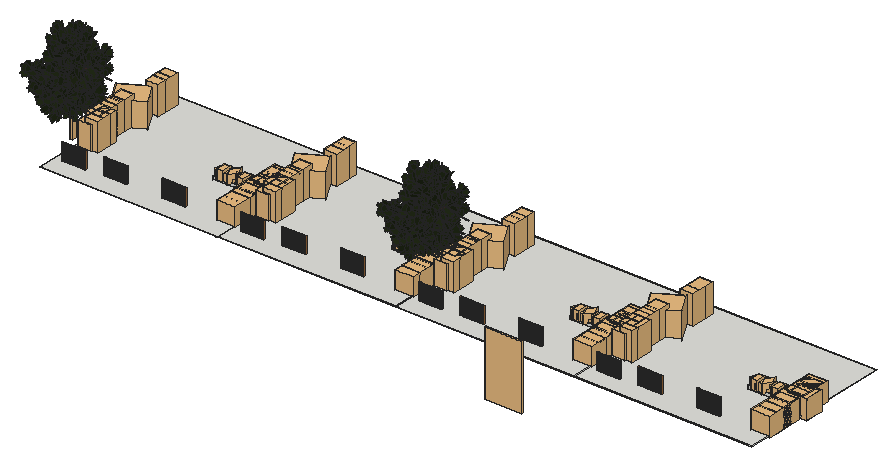
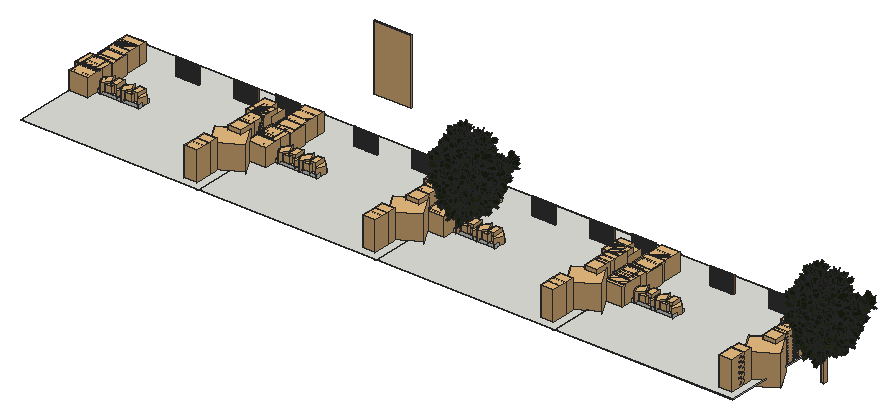
# SketchUp Ruby script. Lengths in inches.
U = 1.inch
M = Sketchup.active_model
def pt(a) = Geom::Point3d.new(a.map { |v| v * U })
def face(e, loops, mat)
  f = e.add_face(loops[0].map { |a| pt(a) })
  loops[1..].each { |l| e.add_face(l.map { |a| pt(a) }).erase! }
  f.material = f.back_material = mat if mat
  f
end
# faces: each face lists its corners as indices into pts; further lists are holes
def faces(e, pts, list, mat = nil) = list.each { |f| face(e, (f[0].is_a?(Array) ? f : [f]).map { |l| l.map { |i| pts[i] } }, mat) }
# xy, xz, yz: faces in a plane at the given z, y or x. An outline is a flat list of corners, or four numbers for a rectangle; further outlines are holes
def ring(l) = l.size == 4 ? [[l[0], l[1]], [l[2], l[1]], [l[2], l[3]], [l[0], l[3]]] : l.each_slice(2).to_a
def flat(e, list, mat, &to3) = list.each { |f| face(e, (f[0].is_a?(Array) ? f : [f]).map { |l| ring(l).map { |u, v| to3.(u, v) } }, mat) }
def xy(e, z, list, mat = nil) = flat(e, list, mat) { |x, y| [x, y, z] }
def xz(e, y, list, mat = nil) = flat(e, list, mat) { |x, z| [x, y, z] }
def yz(e, x, list, mat = nil) = flat(e, list, mat) { |y, z| [x, y, z] }
def lines(e, pts, list) = list.each { |a, b| e.add_line(pt(pts[a]), pt(pts[b])) }
# prism: a flat outline (further loops are holes) pulled along v
def prism(e, loops, v, mat = nil)
  f = face(e, loops, mat); d = Geom::Vector3d.new(v.map { |x| x * U })
  f.pushpull(f.normal.samedirection?(d) ? d.length : -d.length)
end
def box(e, o, s, mat = nil) = prism(e, [[o, [o[0] + s[0], o[1], o[2]], [o[0] + s[0], o[1] + s[1], o[2]], [o[0], o[1] + s[1], o[2]]]], [0, 0, s[2]], mat)
def at(x, y, z, deg = 0) = Geom::Transformation.translation(pt([x, y, z])) * Geom::Transformation.rotation(ORIGIN, Z_AXIS, deg.degrees)
def axes(o, x, y, z) = Geom::Transformation.new([*x, 0, *y, 0, *z, 0, *pt(o).to_a, 1])
def part(name) = M.definitions.add(name)
# library, detail: a bought-in or finely detailed component or shape, given as its bounding box
def library(name, o, s) = part(name).tap { |d| box(d.entities, o, s) }
def detail(e, o, s) = box(e.add_group.entities, o, s)
def put(e, d, t, mat = nil) = e.add_instance(d, t).tap { |i| i.material = mat if mat }
def group(e, t, mat = nil) = e.add_group.tap { |g| g.transformation = t; g.material = mat if mat }.entities
root = M.entities
M.materials.add("Green ash – green texture").color = [33, 41, 22]
M.materials.add("Material__1").color = [95, 70, 46]
M.materials.add("[Color_005]").color = [114, 114, 114]
M.materials.add("[Color_D09]").color = [86, 59, 49]
M.materials.add("[Wood Floor Light]").color = [204, 176, 127]
M.materials.add("[Wood Floor]").color = [155, 105, 61]
c1 = part("Component\#13")
xz(c1.entities,0,[[2.54,0,9.87,0.64,10.99,2.07,11.4,3.42,15.13,2.28,14.48,4.31,16.14,5.21,16.14,6.08,19.81,7.28,19.6,9.67,17.45,11.49,17.45,12.16,18.82,14.37,17.48,14.37,14.41,13.66,14.41,15.23,12.5625,17.49,9.84,15.21,8.9,13.85,7.74,13.625,7.35,12.68,6.87,13.02,6.35,12.27,5.92,10.47,4.2,7.42,2.84,6.89,0,2.38,0.07,1.59,2.8125,4.94,3.37,3.59,2.54,3.37,2.12,2.22]],"Green ash – green texture")
c2 = part("Component\#9")
xz(c2.entities,0,[[1.1,0,1.61,0,2.73,1.11,4.34,2.72,5.21,6.36,5.85,7.16,6.35,6.9375,6.85,8.05,8.03,8.05,8.625,9.25,10.11,11.7,9.56,13.83,9.56,15.84,7.83,15.84,6.03,14.37,5.31,16.54,4.4375,17.39,1.45,14.31,0,9.15,1.4,5.18,3.01,6.08,1.98,1.39]],"Green ash – green texture")
c3 = part("Component\#16")
put(c3.entities,c1,axes([0,7.77,0],[1,0,0],[0,0.89571,0.44464],[0,-0.44464,0.89571]))
put(c3.entities,c2,axes([2.15,6.37,5.26],[0.57629,-0.80824,0.12095],[0.79263,0.51673,-0.3236],[0.19905,0.28236,0.93843]))
c4 = part("Component\#10")
put(c4.entities,c3,axes([-4.97,-3.22,4.05],[0.69883,-0.69034,0.18725],[0.53248,0.3273,-0.7806],[0.47759,0.64522,0.59632]))
c5 = part("Component\#11")
put(c5.entities,c4,axes([0,5.2,2.2],[1,0,0],[0,0.90259,0.43051],[0,-0.43051,0.90259]))
c6 = part("leaf group 2")
put(c6.entities,c5,axes([-11.99,4.41,-4.35],[2.22014,-0.82385,1.14017],[1.36501,1.77637,-1.37441],[-0.33979,1.75315,1.92841]))
c7 = part("Component\#18")
put(c7.entities,c6,axes([-5.27,11.65,1.68],[-0.48323,0.10636,-0.43072],[-0.11515,-0.64511,-0.03012],[-0.42845,0.05342,0.49388]))
c8 = part("Component\#17")
xz(c8.entities,0,[[0.64,0,0,0.1875,4.21,2.81,8.59,4.11,12.8,4.11,19.57,2.81,12.8,3.73,8.59,3.73,4.21,2.3125]],"[Color_D09]")
c9 = part("Leafy twig")
put(c9.entities,c7,axes([23.53,12.57,24.85],[0.06536,-0.90475,-0.42089],[0.61791,-0.2945,0.72901],[-0.78353,-0.30772,0.53981]))
put(c9.entities,c7,axes([22.7,12.25,24.83],[-0.47146,-0.89493,0.11311],[0.80135,-0.48549,-0.35888],[0.36776,-0.0521,0.90651]))
put(c9.entities,c7,axes([24.25,0.65,20.83],[0.8253,-0.50372,0.24924],[0.23848,0.71461,0.65749],[-0.51157,-0.48438,0.71194]))
put(c9.entities,c7,axes([23.54,-2.45,18.63],[0.04689,-0.92492,0.3511],[0.72122,-0.28285,-0.64421],[0.71641,0.2674,0.65188]))
put(c9.entities,c7,axes([22.39,16.15,27.04],[-0.5311,-0.82173,0.2419],[0.41574,0.01583,0.89559],[-0.77461,0.50499,0.40813]))
put(c9.entities,c8,axes([22.76,-5.09,13.48],[0,1.66539,0.44624],[-1.72414,0,0],[0,-0.44624,1.66539]))
c10 = part("Component\#12")
p = [[0,0,0.13],[0.41,0.77,0],[4.07,2.79,10.125],[3.73,2.15,10.23],[7.66,4.77,23.875],[7.4,4.27,23.96],
  [8.6875,5.26,35.99],[8.5,4.91,36.05],[8.32,4.9375,46.95],[8.21,4.74,46.98]]
faces(c10.entities,p,[[0,1,2,3],[3,2,4,5],[4,6,7,5],[6,8,9,7]],"[Color_005]")
c11 = part("Leafy twig \#1")
put(c11.entities,c10,axes([3.13,0.17,-0.45],[3.38032,6.88592,0.52481],[-5.85488,3.97559,0.303],[0,-1.35912,3.54524]))
put(c11.entities,c7,axes([0.37,31.375,148.94],[0.47772,0.64064,-1.51139],[2.85768,-0.62659,0.20284],[-0.43926,-3.3797,-0.3241]))
c12 = part("Leafy tree branch")
put(c12.entities,c9,axes([28.11,72.66,46.26],[0.77413,-0.41274,-0.47998],[0.6311,0.56229,0.53435],[0.04934,-0.71657,0.69577]))
put(c12.entities,c9,axes([31.25,3.94,9.17],[0.73236,0.67893,0.05208],[-0.46223,0.55185,-0.69413],[-0.5,0.48428,0.71797]))
put(c12.entities,c9,axes([20.16,84.84,57.95],[0.96628,0.19619,0.16678],[-0.2575,0.73909,0.62245],[-0.00115,-0.6444,0.76469]))
put(c12.entities,c9,axes([30.13,29.18,11.93],[0.86603,0.2796,0.41452],[0,0.82904,-0.55919],[-0.5,0.48428,0.71797]))
put(c12.entities,c9,axes([47.67,28.63,-3.7],[0.1205,-0.71255,0.69119],[0.96646,0.24327,0.08231],[-0.2268,0.65809,0.71797]))
put(c12.entities,c9,axes([48.76,50.64,76.31],[-0.6716,0.46861,-0.57389],[0.01402,0.78248,0.62252],[0.74078,0.41004,-0.53209]))
put(c12.entities,c11,axes([42.34,0,10.34],[0.39368,0,0],[0,0.22544,-0.24092],[0,0.54032,0.50562]))
put(c12.entities,c9,axes([64.51,80.82,101.08],[-0.99604,0.06562,-0.06004],[-0.0106,0.58266,0.81265],[0.08831,0.81006,-0.57966]))
c13 = library("Tree trunk",[-6.35,9.4375,-76.57],[12.56,13.68,315.77])
c14 = part("Leafy tree branch \#2")
put(c14.entities,c9,axes([-3.64,36.17,23.18],[0.95801,0.10249,0.26779],[-0.28581,0.41631,0.86313],[-0.02302,-0.90343,0.42812]))
put(c14.entities,c9,axes([13.16,55.79,39.92],[0.70711,-0.61725,0.34497],[0,0.48786,0.87292],[-0.70711,-0.61725,0.34497]))
put(c14.entities,c11,axes([18.8125,5.17,0.46],[0.25503,0,0],[0,0.20007,-0.0752],[0,0.16866,0.44872]))
put(c14.entities,c9,axes([23.62,-10.17,21.5],[-0.56253,0.81775,0.12181],[0.38738,0.13053,0.91263],[0.73041,0.56057,-0.39021]))
put(c14.entities,c9,axes([45.18,27.18,68.96],[-0.96593,-0.22593,0.12627],[0.12295,0.02876,0.992],[-0.22775,0.97372,0]))
c15 = part("Component\#22")
put(c15.entities,c11,axes([21.47,3.93,0.22],[0.25503,0,0],[0,0.21068,-0.03601],[0,0.08077,0.47252]))
put(c15.entities,c9,axes([-4.05,13.6875,55.34],[0.70711,0.70373,-0.069],[0,0.09758,0.99523],[0.70711,-0.70373,0.069]))
put(c15.entities,c9,axes([6.52,33.54,18.07],[0.92587,-0.37604,0.03687],[0,0.09758,0.99523],[-0.37784,-0.92145,0.09035]))
c16 = part("Leafy tree branch \#1")
put(c16.entities,c9,axes([26.17,74.02,40.56],[0.25882,-0.64004,0.72344],[0,0.74896,0.66262],[-0.96593,-0.1715,0.19384]))
put(c16.entities,c9,axes([6.38,24.03,55.81],[-0.04786,0.8645,-0.50035],[0.15558,0.50126,0.85119],[0.98666,-0.03711,-0.15849]))
put(c16.entities,c11,axes([17.68,0,1.01],[0.32282,0,0],[0,0.21407,-0.16545],[0,0.37107,0.48011]))
put(c16.entities,c9,axes([-9.1875,31.15,28.07],[0.82314,0.37626,-0.42529],[0,0.74896,0.66262],[0.56784,-0.54543,0.61649]))
put(c16.entities,c9,axes([0.54,-12.07,9.94],[0.19622,0.90478,-0.37799],[-0.67396,0.40444,0.61823],[0.71224,0.13344,0.68914]))
put(c16.entities,c9,axes([7.34,9.15,39.57],[0.05153,0.73872,-0.67204],[0.38679,0.60565,0.6954],[0.92072,-0.29578,-0.25452]))
put(c16.entities,c9,axes([36.2,51.23,15.73],[-0.18626,-0.35374,0.91661],[-0.31641,0.90483,0.2849],[-0.93016,-0.23696,-0.28046]))
c17 = part("Tree")
put(c17.entities,c12,axes([-22.29,52.36,216.76],[0.38964,-1.07313,-0.10036],[1.06809,0.37236,0.19631],[-0.13881,-0.14712,1.22884]))
put(c17.entities,c12,axes([59.83,6.78,230.57],[-1.28826,-0.23008,-0.3647],[0.05148,-1.22938,0.51215],[-0.34663,0.55136,1.25774]))
put(c17.entities,c13,axes([-2.16,-18.04,104.22],[1.30157,0,0],[0,1.30157,0],[0,0,1.36111]))
put(c17.entities,c12,axes([-55.8,4.2,115.32],[1.30157,0,0],[0,1.29536,0.19359],[0,-0.26855,1.38538]))
put(c17.entities,c12,axes([5.36,-52.22,156.04],[-0.23532,1.19719,-0.71362],[-1.32974,0,0.39335],[0.40758,0.6912,1.23603]))
put(c17.entities,c14,axes([-20.09,22.57,317.7],[0,-1.33697,0],[1.33697,0,0],[0,0,1.4573]))
put(c17.entities,c12,axes([44.2,-31.84,172.82],[-1.11894,0.85085,0],[-0.85085,-1.11894,0],[0,0,1.53221]))
put(c17.entities,c12,axes([-10.2,63.7,119.93],[0.28716,-1.46366,0],[1.41378,0.27737,0.38604],[-0.41292,-0.08101,1.5704]))
put(c17.entities,c12,axes([-29.03,-40.72,232.79],[0.5211,0.98898,-0.38718],[-1.02974,0.58664,0.11255],[0.35577,0.28216,1.19957]))
put(c17.entities,c12,axes([44.92,21.7,135.38],[-1.05627,-0.44294,0],[0.44294,-1.05627,0],[0,0,1.24847]))
put(c17.entities,c14,axes([-32.94,-0.59,304.82],[1.2814,-0.22825,0],[0.22825,1.2814,0],[0,0,1.41871]))
put(c17.entities,c14,axes([0.6,-31.29,315.98],[0.13082,1.33422,0],[-1.33422,0.13082,0],[0,0,1.46127]))
put(c17.entities,c14,axes([21.3,1.66,315.16],[-1.25722,0.32198,-0.09905],[-0.32539,-1.26867,0.00612],[-0.08719,0.09194,1.40547]))
put(c17.entities,c15,axes([-19,30.84,372.72],[0.65078,-1.12719,0],[1.12719,0.65078,0],[0,0,1.41871]))
put(c17.entities,c15,axes([14.39,-16.125,357],[-0.73695,1.06095,0.15933],[-1.03698,-0.75397,0.2242],[0.29981,0,1.38667]))
put(c17.entities,c16,axes([-5.9,-20.03,270.39],[0,1.47598,0],[-1.4157,0,0.41751],[0.45509,0,1.54311]))
put(c17.entities,c16,axes([-18.4375,22.18,263.88],[0.84243,-1.42226,-0.32685],[1.40385,0.7063,0.64743],[-0.37678,-0.54841,1.68147]))
put(c17.entities,c16,axes([-29.32,4.9,283.41],[1.35363,0,0],[0,1.33841,0.20242],[0,-0.22063,1.45887]))
put(c17.entities,c16,axes([17.31,11.65,257.52],[-1.14969,-0.5642,-0.25322],[0.46017,-1.12719,0.50159],[-0.40066,0.32434,1.3027]))
put(c17.entities,c16,axes([16.3,15.3125,240.45],[-0.98541,-0.85203,0.68095],[1.00747,-1.01506,0.22317],[0.31818,0.5753,1.40228]))
put(c17.entities,c12,axes([-46.75,22.93,206.12],[1.08363,-0.37101,0],[0.37101,1.08363,0],[0,0,1.24847]))
put(c17.entities,c12,axes([41.1,-35.18,99.125],[-1.05556,0.85173,0.25344],[-0.84493,-1.04965,0.12953],[0.39153,-0.09409,1.38106]))
c18 = library("Group\#166",[0,0,0],[185.03,8.78,321.45])
c19 = library("Potted plant pair",[-0.125,-0.11,0],[4.84,5.4,5.74])
c20 = library("Potted broadleaf plant",[-29.7,0,-10.87],[31.67,38.52,72.45])
c21 = part("Group\#98")
box(c21.entities,[0,0,0],[1.57,1.97,82.68])
c22 = part("Group\#103")
put(c22.entities,c21,at(43.7,15.53,3.9375))
put(c22.entities,c21,at(68.9,15.53,3.9375))
put(c22.entities,c21,at(109.84,15.53,3.9375))
put(c22.entities,c21,at(103.54,15.53,3.9375))
put(c22.entities,c21,at(56.3,15.53,3.9375))
put(c22.entities,c21,at(78.35,15.53,3.9375))
put(c22.entities,c21,at(72.05,15.53,3.9375))
put(c22.entities,c21,at(31.1,15.53,3.9375))
put(c22.entities,c21,at(87.8,15.53,3.9375))
put(c22.entities,c21,at(46.85,15.53,3.9375))
put(c22.entities,c21,at(59.45,15.53,3.9375))
put(c22.entities,c21,at(12.2,15.53,3.9375))
put(c22.entities,c21,at(50,15.53,3.9375))
put(c22.entities,c21,at(106.69,15.53,3.9375))
put(c22.entities,c21,at(34.25,15.53,3.9375))
put(c22.entities,c21,at(81.5,15.53,3.9375))
put(c22.entities,c21,at(53.15,15.53,3.9375))
put(c22.entities,c21,at(27.95,15.53,3.9375))
put(c22.entities,c21,at(65.75,15.53,3.9375))
put(c22.entities,c21,at(18.5,15.53,3.9375))
put(c22.entities,c21,at(40.55,15.53,3.9375))
put(c22.entities,c21,at(75.2,15.53,3.9375))
put(c22.entities,c21,at(21.65,15.53,3.9375))
put(c22.entities,c21,at(62.6,15.53,3.9375))
put(c22.entities,c21,at(84.65,15.53,3.9375))
put(c22.entities,c21,at(100.39,15.53,3.9375))
put(c22.entities,c21,at(112.99,15.53,3.9375))
put(c22.entities,c21,at(24.8,15.53,3.9375))
put(c22.entities,c21,at(37.4,15.53,3.9375))
put(c22.entities,c21,at(97.24,15.53,3.9375))
put(c22.entities,c21,at(2.76,15.53,3.9375))
put(c22.entities,c21,at(5.91,15.53,3.9375))
put(c22.entities,c21,at(94.09,15.53,3.9375))
put(c22.entities,c21,at(15.35,15.53,3.9375))
put(c22.entities,c21,at(9.06,15.53,3.9375))
put(c22.entities,c21,at(90.94,15.53,3.9375))
c23 = part("Group\#109")
put(c23.entities,c22,at(0,0,0),"[Wood Floor]")
g1 = group(c23.entities,at(0,14.54,0))
xy(g1,0,[[0,0,118.11,2.95]],"[Wood Floor]")
xy(g1,3.9375,[[2.76,0,115.35,2.95]],"[Wood Floor]")
xy(g1,30.51,[[2.76,0,115.35,0.98]],"[Wood Floor]")
xy(g1,31.5,[[2.76,0,115.35,0.98]],"[Wood Floor]")
xy(g1,42.52,[[116.29,2.17,117.08,2.95]],"[Wood Floor]")
xy(g1,42.76,[[1.1,0,1.89,0.79]],"[Wood Floor]")
xy(g1,47.24,[[116.29,2.17,117.08,2.95]],"[Wood Floor]")
xy(g1,47.48,[[1.1,0,1.89,0.79]],"[Wood Floor]")
xy(g1,58.07,[[2.76,0,115.35,0.98]],"[Wood Floor Light]")
xy(g1,59.06,[[2.76,0,115.35,0.98]],"[Wood Floor]")
xy(g1,86.61,[[2.76,0,115.35,2.95]],"[Wood Floor]")
xy(g1,90.55,[[0,0,118.11,2.95]],"[Wood Floor]")
xz(g1,0,[[2.76,30.51,115.35,31.5],[2.76,58.07,115.35,59.06]],"[Wood Floor Light]")
xz(g1,0,[[[0,0,118.11,90.55],[2.76,3.9375,115.35,86.61],[1.1,42.76,1.89,47.48]]],"[Wood Floor]")
xz(g1,0.79,[[1.1,42.76,1.89,47.48]],"[Wood Floor]")
xz(g1,0.98,[[2.76,30.51,115.35,31.5],[2.76,58.07,115.35,59.06]],"[Wood Floor]")
xz(g1,2.17,[[116.29,42.52,117.08,47.24]],"[Wood Floor]")
xz(g1,2.95,[[[0,0,118.11,90.55],[2.76,3.9375,115.35,86.61],[116.29,42.52,117.08,47.24]]],"[Wood Floor]")
yz(g1,0,[[0,0,2.95,90.55]],"[Wood Floor]")
yz(g1,1.1,[[0,42.76,0.79,47.48]],"[Wood Floor]")
yz(g1,1.89,[[0,42.76,0.79,47.48]],"[Wood Floor]")
yz(g1,2.76,[[0,3.9375,2.95,3.9375,2.95,86.61,0,86.61,0,59.06,0.98,59.06,0.98,58.07,0,58.07,0,31.5,0.98,31.5,0.98,30.51,0,30.51],[0,30.51,0.98,31.5],[0,58.07,0.98,59.06]],"[Wood Floor]")
yz(g1,115.35,[[0,3.9375,0,30.51,0.98,30.51,0.98,31.5,0,31.5,0,58.07,0.98,58.07,0.98,59.06,0,59.06,0,86.61,2.95,86.61,2.95,3.9375],[0,30.51,0.98,31.5],[0,58.07,0.98,59.06]],"[Wood Floor]")
yz(g1,116.29,[[2.17,42.52,2.95,47.24]],"[Wood Floor]")
yz(g1,117.08,[[2.17,42.52,2.95,47.24]],"[Wood Floor]")
yz(g1,118.11,[[0,0,2.95,90.55]],"[Wood Floor]")
p = [[5.91,2.95,86.61],[5.91,2.95,3.9375]]
lines(g1,p,[[0,1]])
c24 = part("Group\#108")
g2 = group(c24.entities,at(0,0,0),"[Wood Floor]")
put(g2,c21,at(43.7,15.53,3.9375))
put(g2,c21,at(68.9,15.53,3.9375))
put(g2,c21,at(109.84,15.53,3.9375))
put(g2,c21,at(103.54,15.53,3.9375))
put(g2,c21,at(56.3,15.53,3.9375))
put(g2,c21,at(78.35,15.53,3.9375))
put(g2,c21,at(72.05,15.53,3.9375))
put(g2,c21,at(31.1,15.53,3.9375))
put(g2,c21,at(87.8,15.53,3.9375))
put(g2,c21,at(46.85,15.53,3.9375))
put(g2,c21,at(59.45,15.53,3.9375))
g3 = group(g2,at(12.2,15.53,3.9375))
box(g3,[0,0,0],[1.57,1.97,82.68])
put(g2,c21,at(50,15.53,3.9375))
put(g2,c21,at(106.69,15.53,3.9375))
put(g2,c21,at(34.25,15.53,3.9375))
put(g2,c21,at(81.5,15.53,3.9375))
put(g2,c21,at(53.15,15.53,3.9375))
put(g2,c21,at(27.95,15.53,3.9375))
put(g2,c21,at(65.75,15.53,3.9375))
put(g2,c21,at(18.5,15.53,3.9375))
put(g2,c21,at(40.55,15.53,3.9375))
put(g2,c21,at(75.2,15.53,3.9375))
put(g2,c21,at(21.65,15.53,3.9375))
put(g2,c21,at(62.6,15.53,3.9375))
put(g2,c21,at(84.65,15.53,3.9375))
put(g2,c21,at(100.39,15.53,3.9375))
put(g2,c21,at(112.99,15.53,3.9375))
put(g2,c21,at(24.8,15.53,3.9375))
put(g2,c21,at(37.4,15.53,3.9375))
put(g2,c21,at(97.24,15.53,3.9375))
put(g2,c21,at(2.76,15.53,3.9375))
g4 = group(g2,at(5.91,15.53,3.9375))
box(g4,[0,0,0],[1.57,1.97,82.68])
put(g2,c21,at(94.09,15.53,3.9375))
put(g2,c21,at(15.35,15.53,3.9375))
put(g2,c21,at(9.06,15.53,3.9375))
put(g2,c21,at(90.94,15.53,3.9375))
g5 = group(c24.entities,at(0,14.54,0))
xy(g5,0,[[0,0,118.11,2.95]],"[Wood Floor]")
xy(g5,3.9375,[[2.76,0,115.35,2.95]],"[Wood Floor]")
xy(g5,30.51,[[2.76,0,115.35,0.98]],"[Wood Floor]")
xy(g5,31.5,[[2.76,0,115.35,0.98]],"[Wood Floor]")
xy(g5,42.19,[[1.12,0,1.91,0.79]],"[Wood Floor]")
xy(g5,42.49,[[116.24,2.17,117.03,2.95]],"[Wood Floor]")
xy(g5,46.92,[[1.12,0,1.91,0.79]],"[Wood Floor]")
xy(g5,47.22,[[116.24,2.17,117.03,2.95]],"[Wood Floor]")
xy(g5,58.07,[[2.76,0,115.35,0.98]],"[Wood Floor Light]")
xy(g5,59.06,[[2.76,0,115.35,0.98]],"[Wood Floor]")
xy(g5,86.61,[[2.76,0,115.35,2.95]],"[Wood Floor]")
xy(g5,90.55,[[0,0,118.11,2.95]],"[Wood Floor]")
xz(g5,0,[[2.76,30.51,115.35,31.5],[2.76,58.07,115.35,59.06]],"[Wood Floor Light]")
xz(g5,0,[[[0,0,118.11,90.55],[2.76,3.9375,115.35,86.61],[1.12,42.19,1.91,46.92]]],"[Wood Floor]")
xz(g5,0.79,[[1.12,42.19,1.91,46.92]],"[Wood Floor]")
xz(g5,0.98,[[2.76,30.51,115.35,31.5],[2.76,58.07,115.35,59.06]],"[Wood Floor]")
xz(g5,2.17,[[116.24,42.49,117.03,47.22]],"[Wood Floor]")
xz(g5,2.95,[[[0,0,118.11,90.55],[2.76,3.9375,115.35,86.61],[116.24,42.49,117.03,47.22]]],"[Wood Floor]")
yz(g5,0,[[0,0,2.95,90.55]],"[Wood Floor]")
yz(g5,1.12,[[0,42.19,0.79,46.92]],"[Wood Floor]")
yz(g5,1.91,[[0,42.19,0.79,46.92]],"[Wood Floor]")
yz(g5,2.76,[[0,3.9375,2.95,3.9375,2.95,86.61,0,86.61,0,59.06,0.98,59.06,0.98,58.07,0,58.07,0,31.5,0.98,31.5,0.98,30.51,0,30.51],[0,30.51,0.98,31.5],[0,58.07,0.98,59.06]],"[Wood Floor]")
yz(g5,115.35,[[0,3.9375,0,30.51,0.98,30.51,0.98,31.5,0,31.5,0,58.07,0.98,58.07,0.98,59.06,0,59.06,0,86.61,2.95,86.61,2.95,3.9375],[0,30.51,0.98,31.5],[0,58.07,0.98,59.06]],"[Wood Floor]")
yz(g5,116.24,[[2.17,42.49,2.95,47.22]],"[Wood Floor]")
yz(g5,117.03,[[2.17,42.49,2.95,47.22]],"[Wood Floor]")
yz(g5,118.11,[[0,0,2.95,90.55]],"[Wood Floor]")
p = [[5.91,2.95,86.61],[5.91,2.95,3.9375]]
lines(g5,p,[[0,1]])
c25 = library("Pot+Plant",[-20.81,-17.08,-0.03],[39.86,39.43,41.33])
c26 = library("Areca palm plant",[0,0,0],[49.1,36.6,54.46])
c27 = library("Group\#18",[-84.69,-90.07,-0.36],[176.51,175.13,171.4])
c28 = library("Group\#130",[-7.34,-1.2,0],[38.67,35.81,49.04])
c29 = library("Group20\#1",[-20.81,-17.08,3.79],[39.86,39.43,37.51])
c30 = library("Group38\#2",[14.01,28.44,-23.43],[18.58,18.32,38.89])
c31 = part("Group\#20")
put(c31.entities,c26,axes([-6.2,158.41,6.08],[0.45017,-0.56191,0],[0.66137,0.52986,0],[0,0,0.72]))
put(c31.entities,c26,axes([-6.2,56.6,6.08],[0.45017,-0.56191,0],[0.66137,0.52986,0],[0,0,0.72]))
put(c31.entities,c27,axes([14.93,193.18,6.05],[-0.04961,-0.08593,0],[0.08593,-0.04961,0],[0,0,0.10522]))
put(c31.entities,c27,axes([17.19,15.79,6.07],[-0.08133,-0.14087,0],[0.14087,-0.08133,0],[0,0,0.1725]))
put(c31.entities,c28,axes([24.9375,191.72,8],[0,0.79,0],[-0.79,0,0],[0,0,0.79]))
put(c31.entities,c27,axes([14.93,91.37,6.05],[-0.04961,-0.08593,0],[0.08593,-0.04961,0],[0,0,0.10522]))
put(c31.entities,c27,axes([17.19,223.04,6.07],[-0.08133,-0.14087,0],[0.14087,-0.08133,0],[0,0,0.1725]))
put(c31.entities,c28,axes([24.9375,89.91,8],[0,0.79,0],[-0.79,0,0],[0,0,0.79]))
put(c31.entities,c29,axes([18.97,79.98,4.77],[0,0.85,0],[-0.85,0,0],[0,0,0.85]))
put(c31.entities,c29,axes([18.97,181.79,4.77],[0,0.85,0],[-0.85,0,0],[0,0,0.85]))
put(c31.entities,c30,axes([-4.1,100.66,28.17],[0.8848,0,0],[0,0.94674,0],[0,0,0.85826]))
put(c31.entities,c27,axes([14.93,173.12,6.05],[-0.04961,-0.08593,0],[0.08593,-0.04961,0],[0,0,0.10522]))
put(c31.entities,c30,axes([-4.1,-1.15,28.17],[0.8848,0,0],[0,0.94674,0],[0,0,0.85826]))
put(c31.entities,c27,axes([14.93,44.05,6.05],[-0.04961,-0.08593,0],[0.08593,-0.04961,0],[0,0,0.10522]))
put(c31.entities,c27,axes([14.93,145.87,6.05],[-0.04961,-0.08593,0],[0.08593,-0.04961,0],[0,0,0.10522]))
put(c31.entities,c27,axes([14.93,71.3,6.05],[-0.04961,-0.08593,0],[0.08593,-0.04961,0],[0,0,0.10522]))
put(c31.entities,c27,axes([17.19,121.23,6.07],[-0.08133,-0.14087,0],[0.14087,-0.08133,0],[0,0,0.1725]))
g6 = group(c31.entities,at(0,0,0))
xy(g6,0,[[0,0,6,234.8],[30,0,36,234.8]])
xy(g6,3,[[6,0,30,234.8]])
xy(g6,7,[[6,5,30,229.8]],"Material__1")
xy(g6,15,[[[0,0,36,234.8],[6,5,30,229.8]]])
xz(g6,0,[[0,0,6,0,6,3,30,3,30,0,36,0,36,15,0,15]])
xz(g6,5,[[6,7,30,15]])
xz(g6,229.8,[[6,7,30,15]])
xz(g6,234.8,[[0,0,0,15,36,15,36,0,30,0,30,3,6,3,6,0]])
yz(g6,0,[[0,0,234.8,15]])
yz(g6,6,[[0,0,234.8,3],[5,7,229.8,15]])
yz(g6,30,[[0,0,234.8,3],[5,7,229.8,15]])
yz(g6,36,[[0,0,234.8,15]])
xy(root,-18.125,[[276.92,393.78,1156.17,1160.85],[1156.87,393.78,2036.12,1160.85],[2036.8125,393.78,2916.0625,1160.85],[2916.76,393.78,3796.01,1160.85]])
xz(root,393.78,[[276.92,-18.125,1156.17,-16.4375],[1156.87,-18.125,2036.12,-16.4375],[2036.8125,-18.125,2916.0625,-16.4375],[2916.76,-18.125,3796.01,-16.4375]])
xz(root,1160.85,[[276.92,-18.125,1156.17,-16.4375],[1156.87,-18.125,2036.12,-16.4375],[2036.8125,-18.125,2916.0625,-16.4375],[2916.76,-18.125,3796.01,-16.4375]])
yz(root,276.92,[[393.78,-18.125,1160.85,-16.4375]])
yz(root,1156.17,[[393.78,-18.125,1160.85,-16.4375]])
yz(root,1156.87,[[393.78,-18.125,1160.85,-16.4375]])
yz(root,2036.12,[[393.78,-18.125,1160.85,-16.4375]])
yz(root,2036.8125,[[393.78,-18.125,1160.85,-16.4375]])
yz(root,2916.0625,[[393.78,-18.125,1160.85,-16.4375]])
yz(root,2916.76,[[393.78,-18.125,1160.85,-16.4375]])
yz(root,3796.01,[[393.78,-18.125,1160.85,-16.4375]])
put(root,c17,at(1925.59,738.46,-83.65))
put(root,c17,at(165.7,738.46,-83.65))
put(root,c18,at(2718.6,87.32,-53.59))
put(root,c19,axes([1990.03,928.8,-50.23],[13.14,-22.75915,0],[22.75915,13.14,0],[0,0,26.28]))
put(root,c19,axes([2869.98,928.8,-50.23],[13.14,-22.75915,0],[22.75915,13.14,0],[0,0,26.28]))
put(root,c19,axes([230.14,928.8,-50.23],[13.14,-22.75915,0],[22.75915,13.14,0],[0,0,26.28]))
put(root,c19,axes([1110.09,928.8,-50.23],[13.14,-22.75915,0],[22.75915,13.14,0],[0,0,26.28]))
put(root,c20,axes([2106.47,616.9375,-25.16],[2,0,0],[0,2,0],[0,0,2]))
put(root,c20,axes([2986.42,616.9375,-25.16],[2,0,0],[0,2,0],[0,0,2]))
put(root,c20,axes([1226.53,616.9375,-25.16],[2,0,0],[0,2,0],[0,0,2]))
put(root,c20,axes([346.58,616.9375,-25.16],[2,0,0],[0,2,0],[0,0,2]))
put(root,c23,at(2266.83,487.8,-30.48))
put(root,c23,at(3146.77,487.8,-30.48))
put(root,c23,at(1386.88,487.8,-30.48))
put(root,c23,at(506.9375,487.8,-30.48))
put(root,c23,at(2069.64,477.66,-30.26))
put(root,c23,at(2949.58,477.66,-30.26))
put(root,c23,at(1189.69,477.66,-30.26))
put(root,c23,at(309.75,477.66,-30.26))
put(root,c20,axes([2111.0625,694.42,-4.94],[2,0,0],[0,2,0],[0,0,2]))
put(root,c20,axes([2111.0625,659.98,-4.94],[2,0,0],[0,2,0],[0,0,2]))
put(root,c20,axes([2136.5625,622.94,-4.94],[2,0,0],[0,2,0],[0,0,2]))
put(root,c20,axes([2136.5625,659.98,-4.94],[2,0,0],[0,2,0],[0,0,2]))
put(root,c20,axes([2111.0625,741.73,-4.94],[2,0,0],[0,2,0],[0,0,2]))
put(root,c20,axes([2111.0625,802.17,-4.94],[2,0,0],[0,2,0],[0,0,2]))
put(root,c20,axes([3016.51,659.98,-4.94],[2,0,0],[0,2,0],[0,0,2]))
put(root,c20,axes([2991.01,694.42,-4.94],[2,0,0],[0,2,0],[0,0,2]))
put(root,c20,axes([2991.01,659.98,-4.94],[2,0,0],[0,2,0],[0,0,2]))
put(root,c20,axes([3016.51,622.94,-4.94],[2,0,0],[0,2,0],[0,0,2]))
put(root,c20,axes([2991.01,741.73,-4.94],[2,0,0],[0,2,0],[0,0,2]))
put(root,c20,axes([2991.01,802.17,-4.94],[2,0,0],[0,2,0],[0,0,2]))
put(root,c20,axes([376.68,659.98,-4.94],[2,0,0],[0,2,0],[0,0,2]))
put(root,c20,axes([351.18,694.42,-4.94],[2,0,0],[0,2,0],[0,0,2]))
put(root,c20,axes([351.18,659.98,-4.94],[2,0,0],[0,2,0],[0,0,2]))
put(root,c20,axes([376.68,622.94,-4.94],[2,0,0],[0,2,0],[0,0,2]))
put(root,c20,axes([1231.12,802.17,-4.94],[2,0,0],[0,2,0],[0,0,2]))
put(root,c20,axes([1231.12,741.73,-4.94],[2,0,0],[0,2,0],[0,0,2]))
put(root,c20,axes([351.18,741.73,-4.94],[2,0,0],[0,2,0],[0,0,2]))
put(root,c20,axes([351.18,802.17,-4.94],[2,0,0],[0,2,0],[0,0,2]))
put(root,c20,axes([1231.12,659.98,-4.94],[2,0,0],[0,2,0],[0,0,2]))
put(root,c20,axes([1231.12,694.42,-4.94],[2,0,0],[0,2,0],[0,0,2]))
put(root,c20,axes([1256.62,659.98,-4.94],[2,0,0],[0,2,0],[0,0,2]))
put(root,c20,axes([1256.62,622.94,-4.94],[2,0,0],[0,2,0],[0,0,2]))
put(root,c24,at(2553.03,490.74,-26.44))
put(root,c24,at(3432.97,490.74,-26.44))
put(root,c24,axes([2829.52,490.74,-26.44],[0.73274,0,0],[0,1,0],[0,0,1]))
put(root,c24,axes([3709.46,490.74,-26.44],[0.73274,0,0],[0,1,0],[0,0,1]))
put(root,c24,at(1673.08,490.74,-26.44))
put(root,c24,at(793.14,490.74,-26.44))
put(root,c24,axes([1949.57,490.74,-26.44],[0.73274,0,0],[0,1,0],[0,0,1]))
put(root,c24,axes([1069.63,490.74,-26.44],[0.73274,0,0],[0,1,0],[0,0,1]))
put(root,c25,axes([2867.05,660.71,-25.84],[2.28,0,0],[0,2.28,0],[0,0,2.28]))
put(root,c25,axes([3747,660.71,-25.84],[2.28,0,0],[0,2.28,0],[0,0,2.28]))
put(root,c25,axes([2900.8125,734.03,-25.84],[2.28,0,0],[0,2.28,0],[0,0,2.28]))
put(root,c25,axes([2900.8125,735.8,-25.84],[2.28,0,0],[0,2.28,0],[0,0,2.28]))
put(root,c25,axes([3780.75,735.8,-25.84],[2.28,0,0],[0,2.28,0],[0,0,2.28]))
put(root,c25,axes([3780.75,734.03,-25.84],[2.28,0,0],[0,2.28,0],[0,0,2.28]))
put(root,c25,axes([1107.16,660.71,-25.84],[2.28,0,0],[0,2.28,0],[0,0,2.28]))
put(root,c25,axes([1987.11,660.71,-25.84],[2.28,0,0],[0,2.28,0],[0,0,2.28]))
put(root,c25,axes([1140.92,735.8,-25.84],[2.28,0,0],[0,2.28,0],[0,0,2.28]))
put(root,c25,axes([1140.92,734.03,-25.84],[2.28,0,0],[0,2.28,0],[0,0,2.28]))
put(root,c25,axes([2020.87,735.8,-25.84],[2.28,0,0],[0,2.28,0],[0,0,2.28]))
put(root,c25,axes([2020.87,734.03,-25.84],[2.28,0,0],[0,2.28,0],[0,0,2.28]))
put(root,c25,axes([2874.76,805.85,-25.28],[2.28,0,0],[0,2.28,0],[0,0,2.28]))
put(root,c25,axes([2874.76,538.88,-25.28],[2.28,0,0],[0,2.28,0],[0,0,2.28]))
put(root,c25,axes([2874.76,580.63,-25.28],[2.28,0,0],[0,2.28,0],[0,0,2.28]))
put(root,c25,axes([2874.76,627.88,-25.28],[2.28,0,0],[0,2.28,0],[0,0,2.28]))
put(root,c25,axes([3754.7,627.88,-25.28],[2.28,0,0],[0,2.28,0],[0,0,2.28]))
put(root,c25,axes([3754.7,538.88,-25.28],[2.28,0,0],[0,2.28,0],[0,0,2.28]))
put(root,c25,axes([3754.7,580.63,-25.28],[2.28,0,0],[0,2.28,0],[0,0,2.28]))
put(root,c25,axes([3754.7,805.85,-25.28],[2.28,0,0],[0,2.28,0],[0,0,2.28]))
put(root,c25,axes([2874.76,787.42,-25.28],[2.28,0,0],[0,2.28,0],[0,0,2.28]))
put(root,c25,axes([2874.76,744.1,-25.28],[2.28,0,0],[0,2.28,0],[0,0,2.28]))
put(root,c25,axes([3754.7,744.1,-25.28],[2.28,0,0],[0,2.28,0],[0,0,2.28]))
put(root,c25,axes([3754.7,787.42,-25.28],[2.28,0,0],[0,2.28,0],[0,0,2.28]))
put(root,c25,axes([1114.87,627.88,-25.28],[2.28,0,0],[0,2.28,0],[0,0,2.28]))
put(root,c25,axes([1114.87,538.88,-25.28],[2.28,0,0],[0,2.28,0],[0,0,2.28]))
put(root,c25,axes([1114.87,580.63,-25.28],[2.28,0,0],[0,2.28,0],[0,0,2.28]))
put(root,c25,axes([1994.8125,580.63,-25.28],[2.28,0,0],[0,2.28,0],[0,0,2.28]))
put(root,c25,axes([1114.87,805.85,-25.28],[2.28,0,0],[0,2.28,0],[0,0,2.28]))
put(root,c25,axes([1994.8125,627.88,-25.28],[2.28,0,0],[0,2.28,0],[0,0,2.28]))
put(root,c25,axes([1994.8125,538.88,-25.28],[2.28,0,0],[0,2.28,0],[0,0,2.28]))
put(root,c25,axes([1994.8125,805.85,-25.28],[2.28,0,0],[0,2.28,0],[0,0,2.28]))
put(root,c25,axes([1114.87,744.1,-25.28],[2.28,0,0],[0,2.28,0],[0,0,2.28]))
put(root,c25,axes([1994.8125,787.42,-25.28],[2.28,0,0],[0,2.28,0],[0,0,2.28]))
put(root,c25,axes([1114.87,787.42,-25.28],[2.28,0,0],[0,2.28,0],[0,0,2.28]))
put(root,c25,axes([1994.8125,744.1,-25.28],[2.28,0,0],[0,2.28,0],[0,0,2.28]))
put(root,c20,axes([2140.05,992.13,-1.03],[2,0,0],[0,2,0],[0,0,2]))
put(root,c20,axes([2140.05,1037.07,-1.03],[2,0,0],[0,2,0],[0,0,2]))
put(root,c20,axes([3019.99,1037.07,-1.03],[2,0,0],[0,2,0],[0,0,2]))
put(root,c20,axes([3019.99,992.13,-1.03],[2,0,0],[0,2,0],[0,0,2]))
put(root,c20,axes([380.16,1037.07,-1.03],[2,0,0],[0,2,0],[0,0,2]))
put(root,c20,axes([1260.1,992.13,-1.03],[2,0,0],[0,2,0],[0,0,2]))
put(root,c20,axes([380.16,992.13,-1.03],[2,0,0],[0,2,0],[0,0,2]))
put(root,c20,axes([1260.1,1037.07,-1.03],[2,0,0],[0,2,0],[0,0,2]))
put(root,c31,axes([2852.62,739.72,-22.51],[0,1.74,0],[-1,0,0],[0,0,1.23]))
put(root,c31,axes([3732.56,739.72,-22.51],[0,1.74,0],[-1,0,0],[0,0,1.23]))
put(root,c31,axes([1972.67,739.72,-22.51],[0,1.74,0],[-1,0,0],[0,0,1.23]))
put(root,c31,axes([1092.73,739.72,-22.51],[0,1.74,0],[-1,0,0],[0,0,1.23]))
